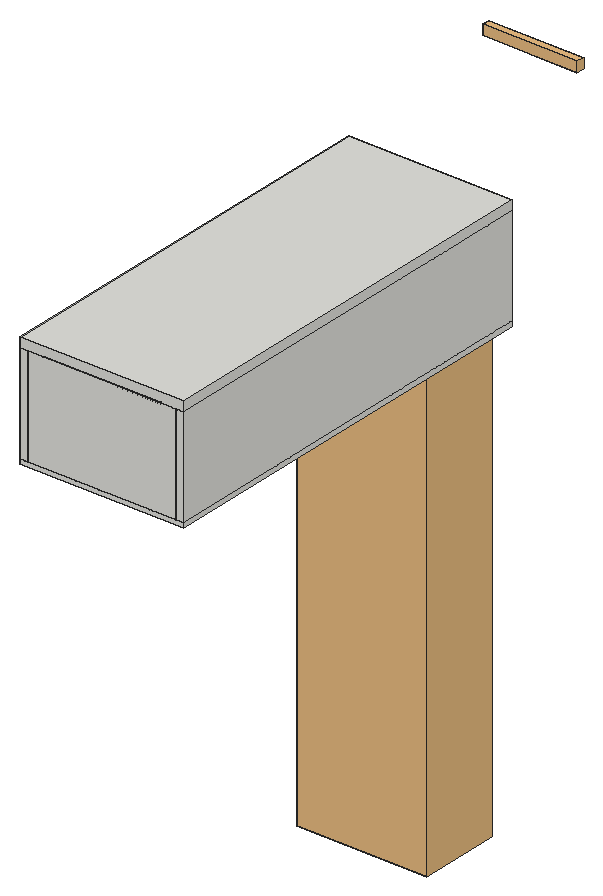
# SketchUp Ruby script. Lengths in inches.
U = 1.inch
M = Sketchup.active_model
def pt(a) = Geom::Point3d.new(a.map { |v| v * U })
def face(e, loops, mat)
  f = e.add_face(loops[0].map { |a| pt(a) })
  loops[1..].each { |l| e.add_face(l.map { |a| pt(a) }).erase! }
  f.material = f.back_material = mat if mat
  f
end
# faces: each face lists its corners as indices into pts; further lists are holes
def faces(e, pts, list, mat = nil) = list.each { |f| face(e, (f[0].is_a?(Array) ? f : [f]).map { |l| l.map { |i| pts[i] } }, mat) }
# xy, xz, yz: faces in a plane at the given z, y or x. An outline is a flat list of corners, or four numbers for a rectangle; further outlines are holes
def ring(l) = l.size == 4 ? [[l[0], l[1]], [l[2], l[1]], [l[2], l[3]], [l[0], l[3]]] : l.each_slice(2).to_a
def flat(e, list, mat, &to3) = list.each { |f| face(e, (f[0].is_a?(Array) ? f : [f]).map { |l| ring(l).map { |u, v| to3.(u, v) } }, mat) }
def xy(e, z, list, mat = nil) = flat(e, list, mat) { |x, y| [x, y, z] }
def xz(e, y, list, mat = nil) = flat(e, list, mat) { |x, z| [x, y, z] }
def yz(e, x, list, mat = nil) = flat(e, list, mat) { |y, z| [x, y, z] }
def lines(e, pts, list) = list.each { |a, b| e.add_line(pt(pts[a]), pt(pts[b])) }
# prism: a flat outline (further loops are holes) pulled along v
def prism(e, loops, v, mat = nil)
  f = face(e, loops, mat); d = Geom::Vector3d.new(v.map { |x| x * U })
  f.pushpull(f.normal.samedirection?(d) ? d.length : -d.length)
end
def box(e, o, s, mat = nil) = prism(e, [[o, [o[0] + s[0], o[1], o[2]], [o[0] + s[0], o[1] + s[1], o[2]], [o[0], o[1] + s[1], o[2]]]], [0, 0, s[2]], mat)
def at(x, y, z, deg = 0) = Geom::Transformation.translation(pt([x, y, z])) * Geom::Transformation.rotation(ORIGIN, Z_AXIS, deg.degrees)
def axes(o, x, y, z) = Geom::Transformation.new([*x, 0, *y, 0, *z, 0, *pt(o).to_a, 1])
def part(name) = M.definitions.add(name)
# library, detail: a bought-in or finely detailed component or shape, given as its bounding box
def library(name, o, s) = part(name).tap { |d| box(d.entities, o, s) }
def detail(e, o, s) = box(e.add_group.entities, o, s)
def put(e, d, t, mat = nil) = e.add_instance(d, t).tap { |i| i.material = mat if mat }
def group(e, t, mat = nil) = e.add_group.tap { |g| g.transformation = t; g.material = mat if mat }.entities
root = M.entities
M.materials.add("Emissive").color = [244, 241, 168]
M.materials.add("Generic").color = [152, 161, 151]
M.materials.add("Generic\#1").color = [218, 213, 213]
M.materials.add("Gold 10k").color = [251, 232, 180]
M.materials.add("Marble White 100cm").color = [222, 222, 222]
M.materials.add("Tiles White 02 160cm").color = [214, 215, 209]
M.materials.add("[Color M07]").color = [58, 58, 58]
M.materials.add("[Wood Floor]").color = [155, 105, 61]
c1 = library("JSilva Jalousie",[-31.89,-0.05,0.1],[63.78,4.97,70.86])
c2 = library("microwave1",[0.56,2.86,0],[17.44,21.22,11.8125])
c3 = library("BERG+Spring+90",[0,0,0],[34.65,15.32,35.9])
c4 = library("PointStove",[0,-0.4,0],[23.23,24.97,35.55])
c5 = library("Bosch Stove",[0,0,0],[36.22,20.12,1.38])
c6 = library("Kitchen sink assembly",[0,0,0],[31.5,19.49,24.78])
c7 = library("frig_samsung",[-10.94,1.57,0],[23.85,23.43,78.74])
c8 = library("Vase 274 001 001",[-4.51,-4.57,0],[9.06,9.12,6.75])
c9 = library("Philodendron moonlight 001",[-12.18,-14.54,0],[24.39,25.11,27.6875])
c10 = library("Vase 014",[-3.77,-3.77,0],[7.54,7.54,8.49])
c11 = library("Peperomia 450 001",[-6.6875,-10.1875,-9.42],[16.7,12.74,19.03])
c12 = library("Apple 73-11",[-5.39,-5.39,0],[10.78,10.78,8.98])
c13 = library("Potted Plant 50-23",[-3.4,-3.5,0],[6.8,7,9.93])
c14 = library("Utensils",[0,-0.54,-0.24],[6.34,6.28,13.37])
c15 = library("Glass_Apothecary_Jar",[-11.5,-3.52,0],[30.82,7.02,10])
c16 = library("ACCESS \#103",[-1.07,0,-1.17],[14.88,24.44,20.18])
c17 = library("kitchen utensils1",[-156.57,0,0],[157.57,98.75,640.76])
c18 = library("DC6",[-214.95,331.04,75.18],[145.41,11.91,20.64])
c19 = library("Pendant 35-41",[-5.93,-5.84,-58.05],[11.88,11.67,58.05])
xy(root,-6,[[0,0,198,498.375]])
xy(root,0,[[0,0,9,0,9,489.375,189,489.375,189,0,198,0,198,498.375,0,498.375],[9,251.223,9,489.375,33,489.375,33,468.5,30.125,468.5,30.125,251.223],[168.6875,309.259,168.6875,468.5,165,468.5,165,489.375,189,489.375,189,309.259],[33,468.5,165,489.375]])
xy(root,0,[[9,0,189,0,189,281.15,173,281.15,173,309.259,168.6875,309.259,168.6875,468.5,30.125,468.5,30.125,251.223,9,251.223]],"Tiles White 02 160cm")
xy(root,4,[[165.75,360.547,168.6875,361.297],[30.125,379.714,32.25,380.114],[30.125,422.545,32.25,422.945],[122.244,466.125,122.644,468.5]])
xy(root,4,[[30.125,251.223,33,294.054],[171,281.15,173,309.259],[30.125,294.054,32.25,294.454],[30.125,294.454,33,336.884],[165,309.259,168.6875,360.547],
  [30.125,336.884,32.25,337.284],[30.125,337.284,33,379.714],[165,361.297,168.6875,412.586],[30.125,380.114,33,422.545],[165.75,412.586,168.6875,413.336],
  [165,413.336,168.6875,468.5],[30.125,422.945,33,465.375],[30.125,465.375,33,468.5],[33,465.375,38.301,468.5],[38.701,465.375,69.552,468.5],
  [69.952,465.375,122.244,468.5],[122.644,465.375,159.732,468.5],[160.132,465.375,165,468.5],[38.301,466.125,38.701,468.5],[69.552,466.125,69.952,468.5],
  [159.732,466.125,160.132,468.5]],"[Wood Floor]")
xy(root,17,[[32.25,294.454,33,336.884],[165,309.259,165.75,360.547],[165,361.297,165.75,412.586],[69.952,465.375,122.244,466.125]],"Gold 10k")
xy(root,17.002,[[32.25,337.284,33,379.714]],"Gold 10k")
xy(root,17.5,[[171,281.15,171.75,309.259]],"Gold 10k")
xy(root,18,[[32.25,294.454,33,336.884],[165,309.259,165.75,360.547],[165,361.297,165.75,412.586],[69.952,465.375,122.244,466.125]],"Gold 10k")
xy(root,18.002,[[32.25,337.284,33,379.714]],"Gold 10k")
xy(root,18.5,[[171,281.15,171.75,309.259]],"Gold 10k")
xy(root,24,[[165,361.297,165.75,412.586]],"Gold 10k")
xy(root,24.001,[[32.25,337.284,33,379.714]],"Gold 10k")
xy(root,25,[[165,361.297,165.75,412.586]],"Gold 10k")
xy(root,25.001,[[32.25,337.284,33,379.714]],"Gold 10k")
xy(root,29.18,[[171,281.15,171.75,309.259]],"Gold 10k")
xy(root,30.18,[[171,281.15,171.75,309.259]],"Gold 10k")
xy(root,31.18,[[171,282.15,183,308.259]])
xy(root,32,[[32.25,422.945,33,465.375],[33,465.375,38.301,466.125]])
xy(root,32,[[32.25,251.223,33,294.054],[32.25,294.454,33,336.884],[165,309.259,165.75,360.547],[32.25,337.284,33,379.714],[165,361.297,165.75,412.586],
  [32.25,380.114,33,422.545],[165,413.336,165.75,466.125],[38.701,465.375,69.552,466.125],[69.952,465.375,122.244,466.125],[122.644,465.375,159.732,466.125],
  [160.132,465.375,165,466.125]],"Gold 10k")
xy(root,33,[[9,251.223,32.25,251.223,32.25,465.375,33,465.375,33,489.375,9,489.375],[165.75,309.259,165.75,466.125,165,466.125,165,489.375,189,489.375,189,309.259],[[33,466.125,165,489.375],[83.797,468.979,97.401,486.243]]])
xy(root,33,[[32.25,251.223,33,465.375],[165,309.259,165.75,466.125],[33,465.375,165,466.125]],"Gold 10k")
xy(root,33.3125,[[97.401,468.979,165,489.375,33,489.375,83.797,486.243,97.401,486.243]])
xy(root,34,[[9,251.223,33,489.375],[165,309.259,189,489.375]])
xy(root,34,[[33,251.223,35,465.375],[163,309.259,165,463.375],[35,463.375,165,465.375]],"Marble White 100cm")
xy(root,36,[[[35,463.375,165,463.375,165,489.375,33,489.375,33,465.375,35,465.375],[83.797,468.979,97.401,486.243]]])
xy(root,36,[[9,251.223,35,251.223,35,465.375,33,465.375,33,489.375,9,489.375,9,262.246,25,262.246,25,259.683,9,259.683],[163,309.259,189,309.259,189,489.375,165,489.375,165,463.375,163,463.375]],"Marble White 100cm")
xy(root,44.976,[[56.066,489.375,140.441,498.375]])
xy(root,52.879,[[9.795,257.121,23.107,259.683]],"Emissive")
xy(root,52.879,[[9,240.375,9,259.683,9.795,259.683,9.795,257.121,23.107,257.121,23.107,259.683,25,259.683,25,240.375]],"[Wood Floor]")
xy(root,54.375,[[171,282.15,183,308.259]])
xy(root,54.653,[[9,240.375,25,259.683]],"[Wood Floor]")
xy(root,55.375,[[171,281.15,171.75,309.259]])
xy(root,56.375,[[171,281.15,171.75,309.259]],"Gold 10k")
xy(root,60,[[186.75,309.259,189,489.375],[9,388.923,10,473.375],[9,473.375,10,489.375],[152.953,487.375,173,489.375],[173,487.375,186.75,489.375],
  [10,487.6875,43.625,489.375]],"Emissive")
xy(root,60,[[173,309.259,186.75,487.375],[10,388.923,25,473.375],[10,473.375,43.625,487.6875],[152.953,473.375,173,487.375]],"[Wood Floor]")
xy(root,60.812,[[24.25,430.399,25,431.149]])
xy(root,61,[[173,390.917,173.75,391.317],[173,418.27,173.75,418.67],[173,445.622,173.75,446.022]])
xy(root,61,[[173,310.259,185,335.611],[173,337.611,185,362.964],[26,473.375,42.625,485.375],[153.953,473.375,172,485.375]],"[Wood Floor]")
xy(root,68.691,[[9.795,257.121,23.107,259.683]],"Emissive")
xy(root,68.691,[[9,240.375,9,259.683,9.795,259.683,9.795,257.121,23.107,257.121,23.107,259.683,25,259.683,25,240.375]],"[Wood Floor]")
xy(root,70.465,[[9,240.375,25,259.683]],"[Wood Floor]")
xy(root,72.629,[[153.953,483.5,172,485.375]],"Emissive")
xy(root,72.629,[[153.953,474.5625,172,483.5]],"[Wood Floor]")
xy(root,72.993,[[184.125,310.259,185,335.611],[183.875,337.611,185,362.964]],"Emissive")
xy(root,72.993,[[173.5625,310.259,184.125,335.611],[173.5625,337.611,183.875,362.964]],"[Wood Floor]")
xy(root,73.699,[[153.953,474.5625,172,485.375]],"[Wood Floor]")
xy(root,74.441,[[26,483.9375,42.625,485.375]],"Emissive")
xy(root,74.441,[[26,473.8125,42.625,483.9375]],"[Wood Floor]")
xy(root,74.53,[[173.5625,310.259,185,335.611],[173.5625,337.611,185,362.964]],"[Wood Floor]")
xy(root,74.75,[[171,240.375,189,281.15]])
xy(root,75.215,[[26,473.8125,42.625,485.375]],"[Wood Floor]")
xy(root,75.75,[[171,274.817,171.75,275.567]],"Gold 10k")
xy(root,75.788,[[56.066,489.375,140.441,498.375]])
xy(root,77.566,[[43.625,487.8125,152.953,489.375]],"Emissive")
xy(root,77.566,[[43.625,473.375,152.953,487.8125]],"[Wood Floor]")
xy(root,78.441,[[43.625,473.375,44.1875,489.375],[152.328,473.375,152.953,489.375]])
xy(root,78.441,[[44.1875,473.375,152.328,489.375]],"[Wood Floor]")
xy(root,79.75,[[10,262.246,10,388.923,24.25,388.923,24.25,388.173,25,388.173,25,346.698,24.25,346.698,24.25,345.948,25,345.948,25,304.472,24.25,304.472,24.25,303.722,25,303.722,25,262.246]])
xy(root,79.75,[[9,262.246,10,388.923]],"Emissive")
xy(root,83.941,[[9.795,257.121,23.107,259.683]],"Emissive")
xy(root,83.941,[[9,240.375,9,259.683,9.795,259.683,9.795,257.121,23.107,257.121,23.107,259.683,25,259.683,25,240.375]],"[Wood Floor]")
xy(root,85.629,[[153.953,484.5625,172,485.375]],"Emissive")
xy(root,85.629,[[153.953,474.5625,172,484.5625]],"[Wood Floor]")
xy(root,85.715,[[9,240.375,25,259.683]],"[Wood Floor]")
xy(root,86.681,[[183.75,310.259,185,335.611],[183.6875,337.611,185,362.964]],"Emissive")
xy(root,86.681,[[173.5625,310.259,183.75,335.611],[173.5625,337.611,183.6875,362.964]],"[Wood Floor]")
xy(root,86.699,[[153.953,474.5625,172,485.375]],"[Wood Floor]")
xy(root,87.129,[[44.1875,487.5625,152.328,489.375]],"Emissive")
xy(root,87.129,[[44.1875,473.375,152.328,487.5625]],"[Wood Floor]")
xy(root,87.191,[[26,483.8125,42.625,485.375]],"Emissive")
xy(root,87.191,[[26,473.8125,42.625,483.8125]],"[Wood Floor]")
xy(root,87.566,[[43.625,473.375,44.1875,489.375],[44.1875,473.375,80.068,473.375,80.068,474.125,80.468,474.125,80.468,473.375,116.51,473.375,116.51,474.125,116.91,474.125,116.91,473.375,152.578,473.375,152.578,489.375,44.1875,489.375],[152.578,473.375,152.953,489.375]])
xy(root,87.566,[[80.068,473.375,80.468,474.125],[116.51,473.375,116.91,474.125]],"Gold 10k")
xy(root,88.09,[[26,473.8125,42.625,485.375]],"[Wood Floor]")
xy(root,88.217,[[173.5625,310.259,185,335.611],[173.5625,337.611,185,362.964]],"[Wood Floor]")
xy(root,92.593,[[171,274.817,171.75,275.567]],"Gold 10k")
xy(root,94.593,[[171,274.817,171.75,275.567]],"Gold 10k")
xy(root,101,[[183.75,310.259,185,335.611],[184.0625,337.611,185,362.964],[153.953,483.875,172,485.375],[26,484.25,42.625,485.375]],"Emissive")
xy(root,101,[[171,274.817,171.75,275.567]],"Gold 10k")
xy(root,101,[[173,310.259,183.75,335.611],[173,337.611,184.0625,362.964],[26,473.375,42.625,484.25],[153.953,473.375,172,483.875]],"[Wood Floor]")
xy(root,102,[[9,259.683,25,262.246],[9,262.246,9,489.375,27,489.375,27,473.375,25,473.375,25,431.149,24.25,431.149,24.25,430.399,25,430.399,25,388.923,24.25,388.923,24.25,388.173,25,388.173,25,346.698,24.25,346.698,24.25,345.948,25,345.948,25,304.472,24.25,304.472,24.25,303.722,25,303.722,25,262.246],[171,309.259,171,471.375,173,471.375,173,446.022,173.75,446.022,173.75,445.622,173,445.622,173,418.67,173.75,418.67,173.75,418.27,173,418.27,173,391.317,173.75,391.317,173.75,390.917,173,390.917,173,309.259],[173,309.259,189,309.259,189,471.375,173,471.375,173,446.022,173.75,446.022,173.75,445.622,173,445.622,173,418.67,173.75,418.67,173.75,418.27,173,418.27,173,391.317,173.75,391.317,173.75,390.917,173,390.917],[27,471.375,27,473.375,80.068,473.375,80.068,474.125,80.468,474.125,80.468,473.375,116.51,473.375,116.51,474.125,116.91,474.125,116.91,473.375,173,473.375,173,471.375],
  [173,471.375,189,489.375],[27,473.375,43.625,489.375],[43.625,473.375,43.625,489.375,173,489.375,173,473.375,116.91,473.375,116.91,474.125,116.51,474.125,116.51,473.375,80.468,473.375,80.468,474.125,80.068,474.125,80.068,473.375]])
xy(root,102,[[9.795,257.121,23.107,259.683]],"Emissive")
xy(root,102,[[9,240.375,9,259.683,9.795,259.683,9.795,257.121,23.107,257.121,23.107,259.683,25,259.683,25,303.722,24.25,303.722,24.25,304.472,25,304.472,25,345.948,24.25,345.948,24.25,346.698,25,346.698,25,388.173,24.25,388.173,24.25,388.923,25,388.923,25,430.399,24.25,430.399,24.25,431.149,25,431.149,25,473.375,27,473.375,27,395.125,26.25,395.125,26.25,394.375,27,394.375,27,318.125,26.25,318.125,26.25,317.375,27,317.375,27,240.375]],"[Wood Floor]")
xy(root,106.875,[[171,240.375,171.75,471.375]],"Gold 10k")
xy(root,107.625,[[171.75,240.375,189,471.375]])
xy(root,107.625,[[171,240.375,171.75,471.375]],"Gold 10k")
xy(root,109.3125,[[27,471.375,171,472.125]],"Gold 10k")
xy(root,110.0625,[[171,471.375,171,472.125,27,472.125,27,489.375,189,489.375,189,471.375]])
xy(root,110.0625,[[27,471.375,171,472.125]],"Gold 10k")
xy(root,120,[[0,0,0,498.375,198,498.375,198,0,189,0,189,489.375,9,489.375,9,0],[9,0,27,240.375],[27,0,171,124.75],[171,0,189,240.375],[27,124.75,171,240.792],
  [9,240.375,9,489.375,27,489.375,27,395.125,26.25,395.125,26.25,394.375,27,394.375,27,318.125,26.25,318.125,26.25,317.375,27,317.375,27,240.375],[171,240.375,189,471.375],[[27,240.792,27,317.375,26.25,317.375,26.25,318.125,27,318.125,27,394.375,26.25,394.375,26.25,395.125,27,395.125,27,471.375,171,471.375,171,240.792],[45.789,259.581,152.211,452.586]],[27,471.375,189,489.375]])
xy(root,121.4375,[[27,0,171,124.75],[27,124.75,171,240.792],[[27,240.792,171,240.792,171,471.375,27,471.375,27,395.125,26.25,395.125,26.25,394.375,27,394.375,27,318.125,26.25,318.125,26.25,317.375,27,317.375],[45.789,259.581,152.211,452.586]]])
xy(root,122.875,[[45.789,259.581,152.211,452.586]])
xy(root,132,[[0,0,198,498.375]])
xz(root,0,[[0,-6,198,0],[0,0,9,120],[9,0,189,120],[189,0,198,120],[0,120,27,120,27,121.4375,171,121.4375,171,120,198,120,198,132,0,132],
  [27,120,171,121.4375]])
xz(root,124.75,[[27,120,171,121.4375]])
xz(root,240.375,[[171,74.75,189,106.875],[171.75,106.875,189,107.625],[171,107.625,189,120]])
xz(root,240.375,[[9,52.879,25,54.653],[9,68.691,25,70.465],[9,83.941,25,85.715],[9,102,27,120]],"[Wood Floor]")
xz(root,240.792,[[27,120,171,121.4375]])
xz(root,251.223,[[9,33,33,34]],"Generic")
xz(root,251.223,[[9,34,35,36]],"Marble White 100cm")
xz(root,251.223,[[9,0,30.125,0,30.125,4,33,4,33,32,32.25,32,32.25,33,9,33]],"[Wood Floor]")
xz(root,259.581,[[45.789,120,152.211,121.4375]])
xz(root,259.581,[[45.789,121.4375,152.211,122.875]],"Emissive")
xz(root,259.683,[[9,52.879,25,54.653],[9,68.691,25,70.465],[9,83.941,25,85.715]])
xz(root,259.683,[[9,36,25,52.879],[9,54.653,25,68.691],[9,70.465,25,83.941],[9,85.715,25,102]],"[Wood Floor]")
xz(root,262.246,[[9,36,25,79.75],[9,79.75,25,102]])
xz(root,274.817,[[171,75.75,171.75,92.593],[171,94.593,171.75,101]],"Gold 10k")
xz(root,275.567,[[171,75.75,171.75,92.593],[171,94.593,171.75,101]],"Gold 10k")
xz(root,281.15,[[173,0,189,0,189,74.75,171,74.75,171,56.375,171.75,56.375,171.75,55.375,171,55.375,171,30.18,171.75,30.18,171.75,29.18,171,29.18,171,18.5,171.75,18.5,171.75,17.5,171,17.5,171,4,173,4]])
xz(root,282.15,[[171,31.18,183,54.375]])
xz(root,294.054,[[32.25,4,33,32]],"Gold 10k")
xz(root,294.454,[[32.25,4,33,17],[32.25,18,33,32]],"Gold 10k")
xz(root,303.722,[[24.25,79.75,25,102]],"Gold 10k")
xz(root,304.472,[[24.25,79.75,25,102]],"Gold 10k")
xz(root,308.259,[[171,31.18,183,54.375]])
xz(root,309.259,[[173,0,189,33],[171,4,171,17.5,171.75,17.5,171.75,18.5,171,18.5,171,29.18,171.75,29.18,171.75,30.18,171,30.18,171,33,173,33,173,4],[171,33,173,34],[173,33,189,34],[171,34,173,36],
  [173,34,189,36],[171,36,171,55.375,171.75,55.375,171.75,56.375,171,56.375,171,102,173,102,173,36],[173,36,189,60],[173,60,189,102]])
xz(root,309.259,[[165,33,171,34],[163,34,171,36]],"Marble White 100cm")
xz(root,309.259,[[168.6875,0,173,0,173,4,171,4,171,17.5,171.75,17.5,171.75,18.5,171,18.5,171,29.18,171.75,29.18,171.75,30.18,171,30.18,171,33,165.75,33,165.75,32,165,32,165,18,165.75,18,165.75,17,165,17,165,4,168.6875,4]],"[Wood Floor]")
xz(root,310.259,[[173.5625,72.993,185,74.53],[173.5625,86.681,185,88.217]])
xz(root,310.259,[[173,61,173,101,185,101,185,88.217,173.5625,88.217,173.5625,86.681,185,86.681,185,74.53,173.5625,74.53,173.5625,72.993,185,72.993,185,61]],"[Wood Floor]")
xz(root,317.375,[[26.25,120,27,121.4375]])
xz(root,317.375,[[26.25,102,27,120]],"Gold 10k")
xz(root,318.125,[[26.25,120,27,121.4375]])
xz(root,318.125,[[26.25,102,27,120]],"Gold 10k")
xz(root,335.611,[[173.5625,72.993,185,74.53],[173.5625,86.681,185,88.217]])
xz(root,335.611,[[173,61,185,61,185,72.993,173.5625,72.993,173.5625,74.53,185,74.53,185,86.681,173.5625,86.681,173.5625,88.217,185,88.217,185,101,173,101]],"[Wood Floor]")
xz(root,336.884,[[32.25,4,33,17],[32.25,18,33,32]],"Gold 10k")
xz(root,337.284,[[32.25,4,33,17.002],[32.25,18.002,33,24.001],[32.25,25.001,33,32]],"Gold 10k")
xz(root,337.611,[[173.5625,72.993,185,74.53],[173.5625,86.681,185,88.217]])
xz(root,337.611,[[173,61,173,101,185,101,185,88.217,173.5625,88.217,173.5625,86.681,185,86.681,185,74.53,173.5625,74.53,173.5625,72.993,185,72.993,185,61]],"[Wood Floor]")
xz(root,345.948,[[24.25,79.75,25,102]],"Gold 10k")
xz(root,346.698,[[24.25,79.75,25,102]],"Gold 10k")
xz(root,360.547,[[165,4,165.75,17]])
xz(root,360.547,[[165,18,165.75,32]],"Gold 10k")
xz(root,361.297,[[165,4,165.75,17],[165,18,165.75,24],[165,25,165.75,32]],"Gold 10k")
xz(root,362.964,[[173.5625,72.993,185,74.53],[173.5625,86.681,185,88.217]])
xz(root,362.964,[[173,61,185,61,185,72.993,173.5625,72.993,173.5625,74.53,185,74.53,185,86.681,173.5625,86.681,173.5625,88.217,185,88.217,185,101,173,101]],"[Wood Floor]")
xz(root,379.714,[[32.25,4,33,17.002],[32.25,18.002,33,24.001],[32.25,25.001,33,32]],"Gold 10k")
xz(root,380.114,[[32.25,4,33,32]],"Gold 10k")
xz(root,388.173,[[24.25,79.75,25,102]],"Gold 10k")
xz(root,388.923,[[9,60,25,79.75]],"Generic\#1")
xz(root,388.923,[[24.25,79.75,25,102]],"Gold 10k")
xz(root,390.917,[[173,61,173.75,102]],"Gold 10k")
xz(root,391.317,[[173,61,173.75,102]],"Gold 10k")
xz(root,394.375,[[26.25,102,27,120],[26.25,120,27,121.4375]])
xz(root,395.125,[[26.25,102,27,120],[26.25,120,27,121.4375]])
xz(root,412.586,[[165,4,165.75,17],[165,18,165.75,24],[165,25,165.75,32]],"Gold 10k")
xz(root,413.336,[[165,4,165.75,32]],"Gold 10k")
xz(root,418.27,[[173,61,173.75,102]],"Gold 10k")
xz(root,418.67,[[173,61,173.75,102]],"Gold 10k")
xz(root,422.545,[[32.25,4,33,32]],"Gold 10k")
xz(root,422.945,[[32.25,4,33,32]],"Gold 10k")
xz(root,430.399,[[24.25,60.812,25,102]],"Gold 10k")
xz(root,431.149,[[24.25,60.812,25,102]],"Gold 10k")
xz(root,445.622,[[173,61,173.75,102]],"Gold 10k")
xz(root,446.022,[[173,61,173.75,102]],"Gold 10k")
xz(root,452.586,[[45.789,120,152.211,121.4375]])
xz(root,452.586,[[45.789,121.4375,152.211,122.875]],"Emissive")
xz(root,463.375,[[163,34,165,36]])
xz(root,463.375,[[35,34,163,36]],"Marble White 100cm")
xz(root,465.375,[[33,34,35,36]])
xz(root,465.375,[[33,4,38.301,32],[38.701,4,69.552,32],[69.952,4,122.244,17],[122.644,4,159.732,32],[160.132,4,165,32],
  [69.952,18,122.244,32],[33,33,165,34]],"Generic")
xz(root,465.375,[[32.25,32,33,33]],"Gold 10k")
xz(root,466.125,[[38.301,4,38.701,32],[69.552,4,69.952,32],[122.244,4,122.644,32],[159.732,4,160.132,32],[69.952,17,122.244,18],
  [33,32,165,33],[165,32,165.75,33]],"Gold 10k")
xz(root,468.5,[[30.125,0,33,4],[33,0,165,4],[165,0,168.6875,4]],"[Wood Floor]")
xz(root,468.979,[[83.797,33,97.401,33.3125],[83.797,33.3125,97.401,36]])
xz(root,471.375,[[171,102,189,102,189,107.625,171.75,107.625,171.75,106.875,171,106.875],[171,107.625,189,110.0625],[171,110.0625,189,120],[27,120,171,121.4375]])
xz(root,471.375,[[27,102,171,102,171,106.875,171.75,106.875,171.75,107.625,171,107.625,171,109.3125,27,109.3125]],"Generic\#1")
xz(root,471.375,[[27,110.0625,171,120]],"[Wood Floor]")
xz(root,472.125,[[27,109.3125,171,110.0625]],"Gold 10k")
xz(root,473.375,[[43.625,87.566,80.068,102],[80.468,87.566,116.51,102],[116.91,87.566,152.953,102]],"Generic\#1")
xz(root,473.375,[[[25,60,43.625,102],[26,61,42.625,101]],[[152.953,60,173,102],[153.953,61,172,101]]],"[Color M07]")
xz(root,473.375,[[43.625,77.566,152.953,78.441],[43.625,78.441,44.1875,87.566],[152.328,78.441,152.953,78.441,152.953,87.566,44.1875,87.566,44.1875,87.129,152.328,87.129]],"[Wood Floor]")
xz(root,473.8125,[[26,74.441,42.625,75.215],[26,87.191,42.625,88.09]],"[Wood Floor]")
xz(root,474.125,[[80.068,87.566,80.468,102],[116.51,87.566,116.91,102]],"Gold 10k")
xz(root,474.5625,[[153.953,72.629,172,73.699],[153.953,85.629,172,86.699]],"[Wood Floor]")
xz(root,485.375,[[153.953,72.629,172,73.699],[24.6,73.699,26,74.223],[26,74.441,42.625,75.215],[153.953,85.629,172,86.699],[26,87.191,42.625,88.09]])
xz(root,485.375,[[26,61,42.625,74.441],[153.953,61,172,72.629],[153.953,73.699,172,85.629],[26,75.215,42.625,87.191],[153.953,86.699,172,101],
  [26,88.09,42.625,101]],"[Wood Floor]")
xz(root,486.243,[[83.797,33,97.401,33.3125],[83.797,33.3125,97.401,36]])
xz(root,489.375,[[9,0,33,33],[33,0,165,33],[165,0,189,33],[9,33,33,34],[33,33,165,33.3125],
  [165,33,189,34],[33,33.3125,165,36],[9,34,33,36],[165,34,189,36],[9,60,43.625,102],
  [152.953,60,152.953,77.566,43.625,77.566,43.625,78.441,173,78.441,173,60],[173,60,189,102],[152.953,78.441,152.953,87.566,43.625,87.566,43.625,102,173,102,173,87.566,172.5,87.566,172.5,78.441],[43.625,78.441,44.1875,87.566],[152.328,78.441,152.953,78.441,152.953,87.566,152.578,87.566,152.578,87.129,152.328,87.129],
  [172.5,78.441,173,87.566],[44.1875,87.129,152.578,87.566],[9,102,27,120],[27,102,189,110.0625],[27,110.0625,189,120]])
xz(root,489.375,[[[9,36,189,36,189,60,152.953,60,152.953,77.566,43.625,77.566,43.625,60,9,60],[56.066,44.976,140.441,75.788]]],"Marble White 100cm")
xz(root,489.375,[[44.1875,78.441,152.328,87.129]],"[Wood Floor]")
xz(root,498.375,[[0,-6,198,0],[[0,0,198,120],[56.066,44.976,140.441,75.788]],[0,120,198,132]])
yz(root,0,[[0,-6,498.375,0],[0,0,498.375,120],[0,120,498.375,132]])
yz(root,9,[[251.223,0,489.375,33],[251.223,33,489.375,34],[251.223,34,489.375,36],[259.683,36,262.246,102],[0,52.879,240.375,54.653],
  [240.375,52.879,259.683,54.653],[473.375,60,473.375,79.75,262.246,79.75,262.246,102,489.375,102,489.375,60],[388.923,60,473.375,79.75],[0,68.691,240.375,70.465],[240.375,68.691,259.683,70.465],
  [0,83.941,240.375,85.715],[240.375,83.941,259.683,85.715],[0,102,240.375,120],[240.375,102,489.375,120]])
yz(root,9,[[262.246,36,489.375,36,489.375,60,388.923,60,388.923,79.75,262.246,79.75]],"Marble White 100cm")
yz(root,9,[[0,0,251.223,0,251.223,36,259.683,36,259.683,52.879,0,52.879],[0,54.653,259.683,68.691],[0,70.465,259.683,83.941],[0,85.715,259.683,102]],"[Wood Floor]")
yz(root,24.25,[[430.399,60.812,431.149,102],[303.722,79.75,304.472,102],[345.948,79.75,346.698,102],[388.173,79.75,388.923,102]],"Gold 10k")
yz(root,25,[[388.923,60.812,430.399,102],[431.149,60.812,473.375,102],[262.246,79.75,303.722,102],[304.472,79.75,345.948,102],[346.698,79.75,388.173,102]],"Generic\#1")
yz(root,25,[[388.923,60,473.375,60.812]],"[Color M07]")
yz(root,25,[[259.683,36,262.246,102],[240.375,52.879,259.683,54.653],[240.375,68.691,259.683,70.465],[240.375,83.941,259.683,85.715]],"[Wood Floor]")
yz(root,26,[[473.8125,74.441,485.375,75.215],[473.8125,87.191,485.375,88.09]])
yz(root,26,[[473.375,61,485.375,61,485.375,74.441,473.8125,74.441,473.8125,75.215,485.375,75.215,485.375,87.191,473.8125,87.191,473.8125,88.09,485.375,88.09,485.375,101,473.375,101]],"[Wood Floor]")
yz(root,26.25,[[394.375,102,395.125,120],[317.375,120,318.125,121.4375],[394.375,120,395.125,121.4375]])
yz(root,26.25,[[317.375,102,318.125,120]],"Gold 10k")
yz(root,27,[[471.375,102,489.375,102,489.375,110.0625,472.125,110.0625,472.125,109.3125,471.375,109.3125],[471.375,110.0625,489.375,120],[0,120,124.75,121.4375],[124.75,120,240.792,121.4375],[240.792,120,317.375,121.4375],
  [318.125,120,394.375,121.4375],[395.125,120,471.375,121.4375]])
yz(root,27,[[318.125,102,394.375,120]],"Generic\#1")
yz(root,27,[[240.375,102,317.375,120],[395.125,102,471.375,102,471.375,109.3125,472.125,109.3125,472.125,110.0625,471.375,110.0625,471.375,120,395.125,120]],"[Wood Floor]")
yz(root,30.125,[[251.223,0,468.5,4]],"[Wood Floor]")
yz(root,32.25,[[294.054,4,294.454,32],[336.884,4,337.284,32],[379.714,4,380.114,32],[422.545,4,422.945,32],[294.454,17,336.884,18],
  [337.284,17.002,379.714,18.002],[337.284,24.001,379.714,25.001],[251.223,32,465.375,33]],"Gold 10k")
yz(root,33,[[468.5,0,489.375,0,489.375,33,466.125,33,466.125,32,465.375,32,465.375,4,468.5,4],[465.375,33,465.375,34,489.375,33.3125,489.375,33],[489.375,33.3125,465.375,34,489.375,34],[465.375,34,489.375,36]])
yz(root,33,[[251.223,4,294.054,32],[294.454,4,336.884,17],[337.284,4,379.714,17.002],[380.114,4,422.545,32],[422.945,4,465.375,32],
  [294.454,18,336.884,32],[337.284,18.002,379.714,24.001],[337.284,25.001,379.714,32],[251.223,33,465.375,34]],"Generic")
yz(root,33,[[465.375,32,466.125,33]],"Gold 10k")
yz(root,35,[[463.375,34,465.375,36]])
yz(root,35,[[251.223,34,463.375,36]],"Marble White 100cm")
yz(root,38.301,[[465.375,4,466.125,32]],"Gold 10k")
yz(root,38.701,[[465.375,4,466.125,32]],"Gold 10k")
yz(root,42.625,[[473.8125,74.441,485.375,75.215],[473.8125,87.191,485.375,88.09]])
yz(root,42.625,[[473.375,61,473.375,101,485.375,101,485.375,88.09,473.8125,88.09,473.8125,87.191,485.375,87.191,485.375,75.215,473.8125,75.215,473.8125,74.441,485.375,74.441,485.375,61]],"[Wood Floor]")
yz(root,43.625,[[473.375,77.566,489.375,78.441],[473.375,78.441,489.375,87.566],[473.375,87.566,489.375,102]])
yz(root,43.625,[[473.375,60,489.375,77.566]],"[Wood Floor]")
yz(root,44.1875,[[473.375,87.129,489.375,87.566]])
yz(root,44.1875,[[473.375,78.441,489.375,87.129]],"[Wood Floor]")
yz(root,45.789,[[259.581,120,299.336,121.4375],[299.336,120,376.336,121.4375],[376.336,120,452.586,121.4375]])
yz(root,45.789,[[259.581,121.4375,299.336,122.875],[299.336,121.4375,376.336,122.875],[376.336,121.4375,452.586,122.875]],"Emissive")
yz(root,56.066,[[489.375,44.976,498.375,75.788]])
yz(root,69.552,[[465.375,4,466.125,32]],"Gold 10k")
yz(root,69.952,[[465.375,4,466.125,17],[465.375,18,466.125,32]],"Gold 10k")
yz(root,80.068,[[473.375,87.566,474.125,102]],"Gold 10k")
yz(root,80.468,[[473.375,87.566,474.125,102]],"Gold 10k")
yz(root,83.797,[[468.979,33,486.243,33.3125],[468.979,33.3125,486.243,36]])
yz(root,97.401,[[468.979,33,486.243,33.3125],[468.979,33.3125,486.243,36]])
yz(root,116.51,[[473.375,87.566,474.125,102]],"Gold 10k")
yz(root,116.91,[[473.375,87.566,474.125,102]],"Gold 10k")
yz(root,122.244,[[465.375,4,466.125,17],[465.375,18,466.125,32]],"Gold 10k")
yz(root,122.644,[[465.375,4,466.125,32]],"Gold 10k")
yz(root,140.441,[[489.375,44.976,498.375,75.788]])
yz(root,152.211,[[259.581,120,452.586,121.4375]])
yz(root,152.211,[[259.581,121.4375,452.586,122.875]],"Emissive")
yz(root,152.328,[[473.375,78.441,489.375,87.129]],"[Wood Floor]")
yz(root,152.953,[[473.375,78.441,489.375,87.566]])
yz(root,152.953,[[473.375,60,489.375,77.566]],"[Wood Floor]")
yz(root,153.953,[[474.5625,72.629,485.375,73.699],[474.5625,85.629,485.375,86.699]])
yz(root,153.953,[[473.375,61,485.375,61,485.375,72.629,474.5625,72.629,474.5625,73.699,485.375,73.699,485.375,85.629,474.5625,85.629,474.5625,86.699,485.375,86.699,485.375,101,473.375,101]],"[Wood Floor]")
yz(root,159.732,[[465.375,4,466.125,32]],"Gold 10k")
yz(root,160.132,[[465.375,4,466.125,32]],"Gold 10k")
yz(root,163,[[309.259,34,463.375,36]],"Marble White 100cm")
yz(root,165,[[468.5,0,489.375,0,489.375,33,466.125,33,466.125,32,465.375,32,465.375,4,468.5,4],[465.375,33,489.375,33,489.375,33.3125,465.375,34],[489.375,33.3125,489.375,34,465.375,34],[463.375,34,489.375,36]])
yz(root,165,[[309.259,4,360.547,17],[361.297,4,412.586,17],[413.336,4,465.375,32],[309.259,18,360.547,32],[361.297,18,412.586,24],
  [361.297,25,412.586,32],[309.259,33,465.375,34]],"Generic")
yz(root,165.75,[[360.547,4,361.297,32],[412.586,4,413.336,32],[309.259,17,360.547,18],[361.297,17,412.586,18],[361.297,24,412.586,25],
  [309.259,32,466.125,33]],"Gold 10k")
yz(root,168.6875,[[309.259,0,468.5,4]],"[Wood Floor]")
yz(root,171,[[[281.15,30.18,309.259,55.375],[282.15,31.18,308.259,54.375]],[0,120,124.75,121.4375],[124.75,120,240.792,121.4375],[240.792,120,471.375,121.4375]])
yz(root,171,[[281.15,4,309.259,17.5],[281.15,18.5,309.259,29.18]],"Generic")
yz(root,171,[[281.15,56.375,309.259,74.75],[241.375,75.75,274.817,92.593],[275.567,75.75,308.259,92.593],[240.375,102,471.375,106.875]],"Generic\#1")
yz(root,171,[[471.375,109.3125,472.125,110.0625]],"Gold 10k")
yz(root,171,[[[240.375,74.75,309.259,93.593],[241.375,75.75,308.259,92.593]],[[240.375,93.593,309.259,102],[241.375,94.593,308.259,101]]],"[Color M07]")
yz(root,171,[[241.375,94.593,274.817,101],[275.567,94.593,308.259,101],[240.375,107.625,471.375,120]],"[Wood Floor]")
yz(root,171.75,[[281.15,17.5,309.259,18.5],[281.15,29.18,309.259,30.18],[281.15,55.375,309.259,56.375],[274.817,75.75,275.567,92.593],[274.817,94.593,275.567,101],
  [240.375,106.875,471.375,107.625]],"Gold 10k")
yz(root,172,[[474.5625,72.629,485.375,73.699],[474.5625,85.629,485.375,86.699]])
yz(root,172,[[473.375,61,473.375,101,485.375,101,485.375,86.699,474.5625,86.699,474.5625,85.629,485.375,85.629,485.375,73.699,474.5625,73.699,474.5625,72.629,485.375,72.629,485.375,61]],"[Wood Floor]")
yz(root,173,[[473.375,60,489.375,78.441],[363.964,61,390.917,102],[391.317,61,418.27,102],[418.67,61,445.622,102],[446.022,61,473.375,102],
  [473.375,78.441,489.375,87.566],[473.375,87.566,489.375,102]])
yz(root,173,[[[309.259,60,336.611,102],[310.259,61,335.611,101]],[[336.611,60,363.964,102],[337.611,61,362.964,101]],[363.964,60,473.375,61]],"[Color M07]")
yz(root,173,[[281.15,0,309.259,4]],"[Wood Floor]")
yz(root,173.5625,[[310.259,72.993,335.611,74.53],[337.611,72.993,362.964,74.53],[310.259,86.681,335.611,88.217],[337.611,86.681,362.964,88.217]],"[Wood Floor]")
yz(root,173.75,[[390.917,61,391.317,102],[418.27,61,418.67,102],[445.622,61,446.022,102]],"Gold 10k")
yz(root,183,[[282.15,31.18,308.259,54.375]])
yz(root,185,[[310.259,72.993,335.611,74.53],[337.611,72.993,362.964,74.53],[310.259,86.681,335.611,88.217],[335.611,86.681,337.611,88.217],[337.611,86.681,362.964,88.217]])
yz(root,185,[[310.259,61,335.611,72.993],[337.611,61,362.964,72.993],[310.259,74.53,335.611,86.681],[337.611,74.53,362.964,86.681],[310.259,88.217,335.611,101],
  [337.611,88.217,362.964,101]],"[Wood Floor]")
yz(root,189,[[0,0,281.15,74.75],[281.15,0,309.259,0,309.259,102,471.375,102,471.375,107.625,240.375,107.625,240.375,74.75,281.15,74.75],[309.259,0,489.375,33],[309.259,33,489.375,34],[309.259,34,489.375,36],
  [309.259,60,489.375,102],[0,74.75,240.375,106.875],[471.375,102,489.375,110.0625],[0,106.875,240.375,107.625],[0,107.625,240.375,120],
  [240.375,107.625,471.375,120],[471.375,110.0625,489.375,120]])
yz(root,189,[[309.259,36,489.375,60]],"Marble White 100cm")
yz(root,198,[[0,-6,498.375,0],[0,0,498.375,120],[0,120,498.375,132]])
p = [[33,489.375,33.3125],[33,465.375,34],[83.797,486.243,33.3125],[83.797,468.979,33.3125],[35,465.375,34],[165,465.375,34],
  [97.401,468.979,33.3125],[165,489.375,33.3125],[172.5,489.375,87.566],[172.5,473.375,87.566],[152.578,489.375,87.129],[152.578,473.375,87.129],
  [33,422.945,32],[33,422.945,32.003],[33,337.284,32],[33,337.284,32.003],[33,380.114,32.003],[33,380.114,32]]
faces(root,p,[[0,1,2],[3,2,1],[1,4,5,6,3],[5,7,6]])
lines(root,p,[[8,9],[10,11],[12,13],[14,15],[16,17]])
put(root,c1,axes([98.65,489.42,44.93],[1.3104,0,0],[0,0.91,0],[0,0,0.4277]))
put(root,c2,axes([189,311.78,46.82],[-1,0,0],[0,-1.23034,0],[0,0,0.64]))
put(root,c3,axes([25,284.71,54.98],[0,1.6214,0],[-1,0,0],[0,0,0.69]))
put(root,c4,axes([169.98,308.26,31.07],[0,-1.12399,0],[0.37315,0,0],[0,0,0.44075]))
put(root,c5,axes([30.37,286.99,35.9],[0,1.31,0],[-1.06212,0,0],[0,0,1]))
put(root,c6,at(82.6,467.79,28.55))
put(root,c7,axes([192.53,264.41,0],[0,1.24,0],[-1,0,0],[0,0,0.94933]))
put(root,c8,at(178.61,329.19,74.53))
put(root,c8,at(178.87,330.07,61))
put(root,c9,at(21.52,242.6,0))
put(root,c10,at(38.74,477.14,88.09))
put(root,c10,axes([159.01,479.2,61],[1,0,0],[0,1,0],[0,0,0.81]))
put(root,c11,at(17.94,252.47,85.27,90))
put(root,c12,at(172.73,360.95,36))
put(root,c13,at(17,248.4375,70.51))
put(root,c13,at(16.875,255.27,36))
put(root,c13,at(21.35,425.39,36))
put(root,c13,at(56.79,480.75,36))
put(root,c13,at(142.34,480.13,36))
put(root,c13,at(182.01,339.33,36))
put(root,c13,at(79.22,481.33,78.44))
put(root,c13,at(108.59,479.47,78.44))
put(root,c13,at(179.98,355.68,74.53))
put(root,c13,at(179.3125,330.4,88.22))
put(root,c13,at(176.9,320.0625,61))
put(root,c14,at(15.41,470.62,36))
put(root,c15,axes([55.6875,482.45,78.44],[1,0,0],[0,1,0],[0,0,0.86884]))
put(root,c16,at(185.97,464.15,37.17,172.7))
put(root,c17,at(182.9,387.08,-559.0625))
put(root,c18,at(240.95,145.65,0))
put(root,c13,at(28.44,481.77,88.09))
put(root,c10,axes([168.23,481.61,61],[1,0,0],[0,1,0],[0,0,0.81]))
put(root,c18,axes([136.61,480.99,78.39],[0.79,0,0],[0,0.79,0],[0,0,0.5846]))
put(root,c19,at(94.66,318.04,122.875))
put(root,c8,at(16.4,253.18,54.65))
put(root,c8,at(179.76,355.54,61))
put(root,c13,at(179.3125,352.83,88.22))
